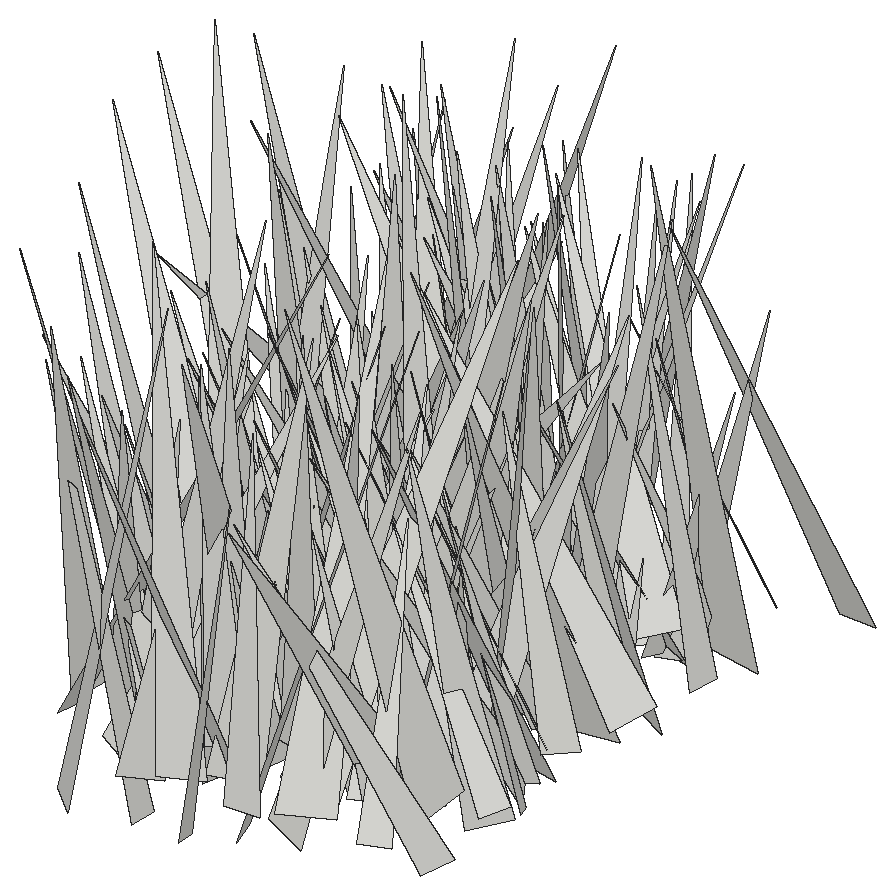
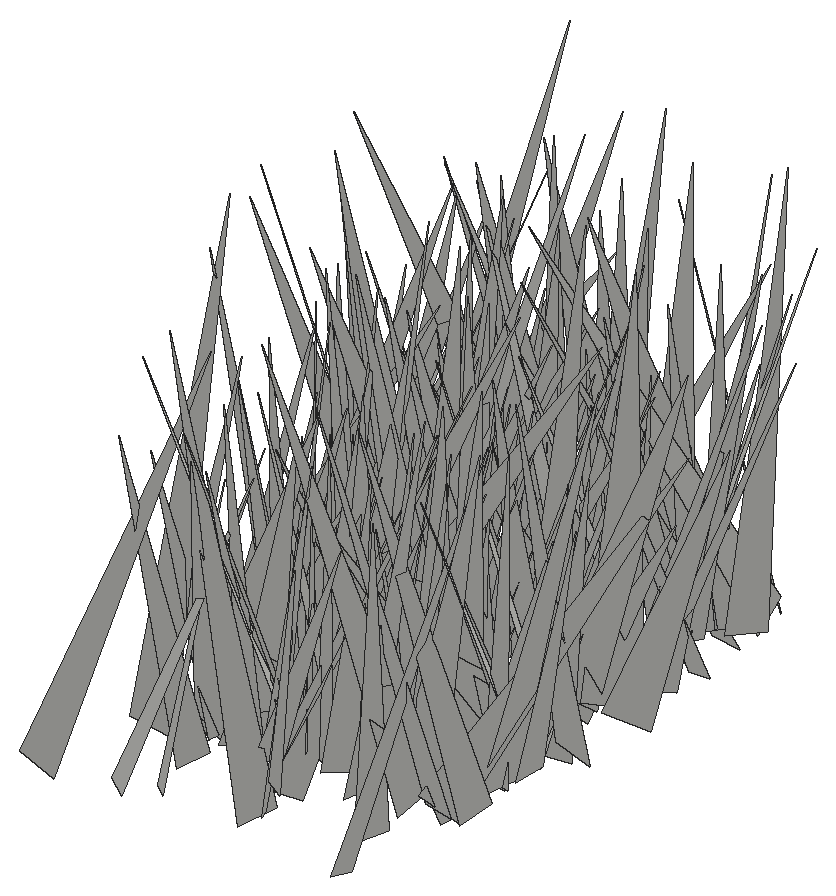
# SketchUp Ruby script. Lengths in inches.
U = 1.inch
M = Sketchup.active_model
def pt(a) = Geom::Point3d.new(a.map { |v| v * U })
def face(e, loops, mat)
  f = e.add_face(loops[0].map { |a| pt(a) })
  loops[1..].each { |l| e.add_face(l.map { |a| pt(a) }).erase! }
  f.material = f.back_material = mat if mat
  f
end
# faces: each face lists its corners as indices into pts; further lists are holes
def faces(e, pts, list, mat = nil) = list.each { |f| face(e, (f[0].is_a?(Array) ? f : [f]).map { |l| l.map { |i| pts[i] } }, mat) }
# xy, xz, yz: faces in a plane at the given z, y or x. An outline is a flat list of corners, or four numbers for a rectangle; further outlines are holes
def ring(l) = l.size == 4 ? [[l[0], l[1]], [l[2], l[1]], [l[2], l[3]], [l[0], l[3]]] : l.each_slice(2).to_a
def flat(e, list, mat, &to3) = list.each { |f| face(e, (f[0].is_a?(Array) ? f : [f]).map { |l| ring(l).map { |u, v| to3.(u, v) } }, mat) }
def xy(e, z, list, mat = nil) = flat(e, list, mat) { |x, y| [x, y, z] }
def xz(e, y, list, mat = nil) = flat(e, list, mat) { |x, z| [x, y, z] }
def yz(e, x, list, mat = nil) = flat(e, list, mat) { |y, z| [x, y, z] }
def lines(e, pts, list) = list.each { |a, b| e.add_line(pt(pts[a]), pt(pts[b])) }
# prism: a flat outline (further loops are holes) pulled along v
def prism(e, loops, v, mat = nil)
  f = face(e, loops, mat); d = Geom::Vector3d.new(v.map { |x| x * U })
  f.pushpull(f.normal.samedirection?(d) ? d.length : -d.length)
end
def box(e, o, s, mat = nil) = prism(e, [[o, [o[0] + s[0], o[1], o[2]], [o[0] + s[0], o[1] + s[1], o[2]], [o[0], o[1] + s[1], o[2]]]], [0, 0, s[2]], mat)
def at(x, y, z, deg = 0) = Geom::Transformation.translation(pt([x, y, z])) * Geom::Transformation.rotation(ORIGIN, Z_AXIS, deg.degrees)
def axes(o, x, y, z) = Geom::Transformation.new([*x, 0, *y, 0, *z, 0, *pt(o).to_a, 1])
def part(name) = M.definitions.add(name)
# library, detail: a bought-in or finely detailed component or shape, given as its bounding box
def library(name, o, s) = part(name).tap { |d| box(d.entities, o, s) }
def detail(e, o, s) = box(e.add_group.entities, o, s)
def put(e, d, t, mat = nil) = e.add_instance(d, t).tap { |i| i.material = mat if mat }
def group(e, t, mat = nil) = e.add_group.tap { |g| g.transformation = t; g.material = mat if mat }.entities
root = M.entities
c1 = part("fur_instance\#9")
p = [[0.8125,0,1.79],[0.67,-0.02,1.48],[0,-0.11,0],[0,0.11,0]]
faces(c1.entities,p,[[0,1,2,3]])
put(root,c1,axes([64.84,118.15,-27.1],[-3.24359,5.98487,0.42852],[5.75195,2.96279,2.1587],[-1.708,-1.38792,6.45597]))
put(root,c1,axes([65.26,123.43,-27.1],[-7.08698,0.49693,1.41438],[0.58095,7.2106,0.37757],[1.38199,-0.48283,7.09434]))
put(root,c1,axes([66.96,118.08,-27.1],[-3.17251,7.14398,0.8627],[6.87917,2.73438,2.65436],[-2.11131,-1.82544,7.35225]))
put(root,c1,axes([65.07,122.26,-27.1],[-4.79431,0.50788,0.77321],[0.45097,4.84644,-0.38709],[0.80772,0.30866,4.80557]))
put(root,c1,axes([65.85,125.42,-27.1],[3.04305,-5.48081,0.27728],[-4.42438,-2.6378,-3.58374],[-3.24669,-1.54241,5.14356]))
put(root,c1,axes([65.59,115.98,-27.1],[-5.22696,-1.19875,0.73288],[-0.94186,5.08442,1.59898],[1.04259,-1.41663,5.11873]))
put(root,c1,axes([65.69,117.69,-27.1],[-4.19179,6.94453,1.88873],[7.18228,4.17546,0.58769],[0.45687,-1.92457,8.09026]))
put(root,c1,axes([64.86,120.54,-27.1],[1.29784,6.7007,1.25957],[6.74597,-1.44798,0.75208],[-0.98888,-1.08363,6.78367]))
put(root,c1,axes([67.71,114.12,-28.22],[-7.51977,-1.08655,0.44758],[-1.14316,7.43533,-1.15625],[0.27218,1.20961,7.50937]))
put(root,c1,axes([67.67,117.16,-28.22],[-1.87407,5.07403,0.37598],[4.58214,1.50899,2.47512],[-2.21159,-1.17322,4.80954]))
put(root,c1,axes([65.07,116.1,-27.1],[-4.32761,-0.50237,2.11035],[0.41917,4.42689,1.9134],[2.12844,-1.89326,3.91401]))
put(root,c1,axes([66.42,113.57,-27.1],[-6.02827,1.48886,1.73676],[1.72693,6.17226,0.7029],[1.50026,-1.12234,6.1695]))
put(root,c1,axes([66.98,121.77,-28.22],[-1.60239,4.56784,1.22355],[4.62571,1.24567,1.40748],[-0.98238,-1.58525,4.63161]))
put(root,c1,axes([66.41,119.52,-28.22],[-2.06507,4.56305,1.47225],[4.79287,1.92061,0.77009],[-0.13147,-1.65628,4.94903]))
put(root,c1,axes([65.53,123.23,-27.1],[1.09401,4.63876,2.44173],[5.21296,-1.22556,-0.00737],[-0.55243,-2.37843,4.76601]))
put(root,c1,axes([67.625,111.83,-27.1],[-5.88104,-3.53705,0.94417],[-3.64814,5.81133,-0.9531],[0.30541,1.30636,6.79625]))
put(root,c1,axes([65.98,115.75,-27.1],[-3.08221,-2.2445,0.63722],[-2.14243,3.14072,0.69983],[0.92405,-0.20483,3.74807]))
put(root,c1,axes([66.2,121.26,-27.1],[3.80784,5.11048,0.67094],[4.57882,-3.73693,2.47721],[-2.36675,0.99257,5.87197]))
put(root,c1,axes([67.18,124.61,-27.1],[-2.59565,5.50063,1.7013],[5.74289,2.3395,1.19781],[-0.41302,-2.03926,5.96319]))
put(root,c1,axes([67.8,111.69,-27.1],[-4.98087,1.16288,0.32288],[1.15979,4.99131,-0.08543],[0.33384,0.00996,5.1141]))
put(root,c1,axes([65.36,112.02,-27.1],[6.33398,-2.31725,1.64534],[-1.9481,-6.46653,-1.60778],[-2.06922,-1.00519,6.55011]))
put(root,c1,axes([66.54,119.98,-28.22],[-3.71629,-3.62879,0.54604],[-3.4741,3.72939,1.13989],[1.18191,-0.44788,5.0675]))
put(root,c1,axes([64.92,114.73,-27.1],[1.35315,4.35582,0.79538],[4.34518,-1.14634,-1.11449],[0.85157,-1.07217,4.42291]))
put(root,c1,axes([66.9,128.53,-28.22],[-6.16239,-2.08969,1.53365],[-1.42213,6.03269,2.50561],[2.16712,-1.98337,6.00531]))
put(root,c1,axes([67.79,117.45,-27.1],[-4.13289,0.76106,0.51137],[0.79822,4.14817,0.27763],[0.45116,-0.36746,4.1932]))
put(root,c1,axes([64.83,125,-27.1],[6.22243,-0.20354,0.93497],[-0.30289,-6.25415,0.65425],[-0.90767,0.69164,6.19128]))
put(root,c1,axes([67.47,124.59,-27.1],[4.90342,0.51596,3.18153],[0.4361,-5.84514,0.27581],[-3.19346,-0.00597,4.92277]))
put(root,c1,axes([68.41,122.6875,-28.22],[-6.24341,4.5177,1.05822],[4.50521,6.32678,-0.4296],[1.11019,-0.26807,7.69449]))
put(root,c1,axes([66.2,112.4,-27.1],[5.00192,-1.81934,1.03799],[-1.65,-5.07776,-0.94895],[-1.29032,-0.55947,5.23724]))
put(root,c1,axes([67.18,119.29,-28.22],[-0.06707,-7.91469,2.47451],[-8.29222,0.04381,-0.08466],[-0.06773,2.47503,7.91452]))
put(root,c1,axes([68.17,126.02,-27.1],[-6.22894,0.57755,1.75246],[0.68588,6.45268,0.31131],[1.71297,-0.48351,6.24791]))
put(root,c1,axes([66.53,112.71,-27.1],[6.05103,1.03829,2.78411],[2.19851,-5.8136,-2.61017],[-1.99898,-3.2509,5.55698]))
put(root,c1,axes([69.5,108.86,-28.22],[-6.22819,-1.34042,0.61243],[-1.44458,6.07908,-1.38568],[0.29149,1.48668,6.21828]))
put(root,c1,axes([68.08,118.91,-28.22],[-5.34659,-1.99732,0.9572],[-1.60106,5.21354,1.93576],[1.5304,-1.52357,5.36919]))
put(root,c1,axes([65.77,125.51,-27.1],[2.77668,6.00015,1.42785],[6.14966,-2.57364,-1.14395],[0.47149,-1.76779,6.51177]))
put(root,c1,axes([67.5625,126.33,-28.22],[-4.75498,1.70819,1.94206],[1.76287,5.11453,-0.18234],[1.89256,-0.47231,5.04921]))
put(root,c1,axes([68.23,116.49,-27.1],[-3.61922,1.27993,0.57976],[1.16278,3.62754,-0.74965],[0.78884,0.52519,3.76496]))
put(root,c1,axes([66.6,112.66,-27.1],[2.66304,-4.00114,1.09323],[-4.14622,-2.60379,0.57024],[-0.11461,1.22768,4.77239]))
put(root,c1,axes([67.33,124.14,-27.1],[-1.25475,3.57203,1.31412],[3.70812,1.4592,-0.42579],[0.858,-1.08261,3.76198]))
put(root,c1,axes([70.04,118.73,-28.22],[-4.54723,-4.75664,0.92618],[-4.80738,4.26788,-1.68375],[-0.61038,1.82216,6.36144]))
put(root,c1,axes([67.2,119.92,-28.22],[3.79033,1.52401,0.8214],[1.29616,-3.80865,1.0854],[-1.14773,0.73179,3.93842]))
put(root,c1,axes([68.78,120.83,-27.1],[3.00603,-4.02582,3.59921],[-4.80148,-3.87769,-0.32715],[-2.47129,2.63706,5.01362]))
put(root,c1,axes([67.25,108.29,-28.22],[4.64173,5.41011,1.53464],[5.42173,-4.8336,0.64123],[-1.49305,-0.73288,7.09956]))
put(root,c1,axes([67.07,113.09,-28.22],[2.82826,-4.43632,2.67471],[-5.15951,-2.68482,1.00262],[-0.46309,2.81866,5.16476]))
put(root,c1,axes([65.51,110.8,-27.1],[7.33228,1.89466,0.16833],[1.78282,-7.07911,2.02191],[-0.66303,1.91751,7.29821]))
put(root,c1,axes([67.9375,118.45,-27.1],[-1.16882,5.10436,1.64073],[5.31118,1.33199,-0.3603],[0.7334,-1.51127,5.22406]))
put(root,c1,axes([68.32,125.61,-28.22],[-5.67591,-0.59927,2.29984],[-0.30227,6.08824,0.84044],[2.35734,-0.66225,5.64524]))
put(root,c1,axes([69.52,119.3125,-27.1],[-0.27528,4.26527,0.41219],[4.05575,0.12601,1.40472],[-1.38323,-0.47937,4.03672]))
put(root,c1,axes([67.23,124.49,-27.1],[1.7878,3.1828,1.34143],[3.44443,-1.53093,-0.95817],[0.2561,-1.62848,3.52255]))
put(root,c1,axes([67.1875,114.24,-28.22],[5.06961,3.19969,0.78256],[3.08145,-5.11429,0.94868],[-1.16407,0.39664,5.91937]))
put(root,c1,axes([72.34,121.27,-27.1],[-3.051,-7.21191,1.32168],[-6.61753,2.09219,-3.8598],[-3.15701,2.58422,6.81338]))
put(root,c1,axes([69.63,111.6,-28.22],[-5.24858,-0.93793,1.2858],[-1.33069,5.01688,-1.77222],[0.87308,2.00792,5.02857]))
put(root,c1,axes([69.12,120.68,-28.22],[-5.6995,-3.45113,0.56108],[-3.05969,5.44221,2.39374],[1.69215,-1.78365,6.21808]))
put(root,c1,axes([67.03,121.89,-27.1],[-1.28039,5.01222,0.36244],[4.5705,1.31696,-2.06622],[2.08908,0.19072,4.74262]))
put(root,c1,axes([68.97,123.79,-27.1],[3.31439,2.62679,2.62231],[3.03004,-3.94532,0.12232],[-2.14367,-1.5153,4.22732]))
put(root,c1,axes([66.57,119.5625,-27.1],[4.70564,3.18962,0.73071],[3.27223,-4.59158,-1.02983],[-0.01227,-1.26267,5.59072]))
put(root,c1,axes([70.63,117.9375,-28.22],[-2.19806,-5.17129,0.07017],[-4.98418,2.09779,-1.52836],[-1.38027,0.66005,5.4072]))
put(root,c1,axes([68.04,121.0625,-28.22],[-4.86484,4.13925,3.64162],[4.78109,5.5858,0.03796],[2.74517,-2.39309,6.38738]))
put(root,c1,axes([66.61,125.52,-27.1],[7.58645,0.4489,1.20084],[0.2907,-7.62155,1.01257],[-1.24861,0.95304,7.53196]))
put(root,c1,axes([69.76,115.34,-28.22],[-6.59248,-1.12335,1.64682],[-1.04061,6.79216,0.46743],[1.70031,-0.1986,6.67115]))
put(root,c1,axes([68.28,120.45,-27.1],[4.10212,-1.60455,0.85508],[-1.23063,-4.00368,-1.60913],[-1.3384,-1.23658,4.10033]))
put(root,c1,axes([66.73,111.22,-28.22],[2.4491,6.4359,0.09226],[6.32974,-2.3903,-1.28384],[1.16776,-0.54137,6.7654]))
put(root,c1,axes([71.85,125.07,-28.22],[-7.66892,-1.90839,0.15613],[-1.91216,7.66661,-0.21311],[0.09999,0.24454,7.89993]))
put(root,c1,axes([70.18,109.5625,-27.1],[-1.69454,7.12423,1.83382],[7.32335,1.45532,1.11334],[-0.69716,-2.02889,7.23786]))
put(root,c1,axes([70.8,117.98,-27.1],[-4.9286,0.63717,0.02707],[0.62924,4.89286,-0.60144],[0.10377,0.59304,4.93308]))
put(root,c1,axes([69.33,108.95,-27.1],[-6.96616,2.88196,1.8212],[2.05018,6.85162,-3.00033],[2.72382,2.21349,6.91601]))
put(root,c1,axes([71.57,110.26,-27.1],[-3.32714,-4.87132,0.7615],[-4.7527,2.92423,-2.05917],[-1.31203,1.7603,5.52806]))
put(root,c1,axes([70.46,123.27,-28.22],[0.69444,-4.60057,1.02449],[-4.36557,-1.0182,-1.61314],[-1.77671,0.70364,4.36409]))
put(root,c1,axes([69.4,125.52,-27.1],[-3.39336,2.50243,2.08506],[2.97495,3.60715,0.51243],[1.32637,-1.68843,4.18502]))
put(root,c1,axes([66.8125,120.625,-28.22],[5.86888,-2.59714,0.14419],[-2.59865,-5.83866,0.60558],[0.11385,0.61201,6.38922]))
put(root,c1,axes([69.11,116.08,-28.22],[3.19373,2.97376,0.94617],[2.91746,-3.32577,0.60507],[-1.10768,-0.18543,4.3217]))
put(root,c1,axes([67.9,114.83,-28.22],[-0.42992,-4.68733,0.89248],[-4.33891,0.75688,1.88505],[1.98531,0.63912,4.31306]))
put(root,c1,axes([72.78,121.91,-27.1],[-6.95314,3.37085,0.59923],[3.40426,6.66259,2.02209],[-0.36434,-2.07731,7.45788]))
put(root,c1,axes([71.16,125.97,-28.22],[3.15853,-4.87453,2.05329],[-4.28659,-3.76007,-2.33247],[-3.09874,0.23284,5.31949]))
put(root,c1,axes([71.38,126.27,-27.1],[-4.19942,1.95994,0.17006],[1.96728,4.18576,0.33862],[0.01038,-0.37878,4.62189]))
put(root,c1,axes([71.82,123.75,-28.22],[-5.34119,3.3335,0.99515],[3.47843,5.14626,1.43085],[0.05516,-1.74201,6.13133]))
put(root,c1,axes([70.14,111.66,-27.1],[1.65081,-5.08845,2.41171],[-5.51574,-1.96719,-0.37505],[-1.13372,2.16141,5.33637]))
put(root,c1,axes([68.52,115.18,-28.22],[7.11754,-4.23376,0.53848],[-3.90576,-6.88369,-2.49681],[-1.7204,-1.88792,7.89621]))
put(root,c1,axes([71.87,122.33,-28.22],[-2.19401,4.08598,0.64459],[3.98986,1.89782,1.55038],[-1.09165,-1.27572,4.37096]))
put(root,c1,axes([70.47,119.62,-27.1],[0.64716,8.27924,1.09317],[8.31403,-0.74193,0.69715],[-0.78591,-1.0312,8.27518]))
put(root,c1,axes([66.4,123.8,-28.22],[2.58062,-5.27777,0.62862],[-4.46822,-1.77579,3.43383],[2.87837,1.97518,4.76689]))
put(root,c1,axes([70.23,127.41,-27.1],[-1.89592,-3.45095,1.30694],[-3.60556,2.04518,0.16982],[0.78554,1.05823,3.9338]))
put(root,c1,axes([69.74,112.5,-27.1],[2.04038,-5.82637,1.87095],[-6.1057,-2.07021,0.21174],[-0.4092,1.83789,6.16967]))
put(root,c1,axes([70.04,125.37,-27.1],[-2.18081,-4.36379,1.96245],[-4.63729,2.45895,0.31456],[1.17875,1.60022,4.86823]))
put(root,c1,axes([71.23,125.05,-28.22],[-3.89073,-3.2521,0.98713],[-3.3181,3.95947,-0.03367],[0.73538,0.65937,5.07078]))
put(root,c1,axes([70.78,119.67,-27.1],[-3.9819,-2.09854,0.99873],[-1.89028,4.07705,1.03024],[1.35209,-0.4803,4.38155]))
put(root,c1,axes([68.3,120.58,-27.1],[3.9818,-4.86666,0.84742],[-4.90357,-3.76221,1.43455],[0.59785,1.55519,6.12218]))
put(root,c1,axes([71.84,122.3,-28.22],[-6.35948,3.06032,1.72749],[3.24757,6.48259,0.47123],[1.34279,-1.18457,7.04176]))
put(root,c1,axes([71.05,124.27,-27.1],[1.22573,-5.85041,2.29876],[-6.17569,-1.55733,-0.67049],[-1.1715,2.08841,5.93971]))
put(root,c1,axes([68.97,114.5,-28.22],[0.04423,5.29855,0.55334],[5.02486,0.14232,-1.76445],[1.76963,-0.53655,4.99632]))
put(root,c1,axes([72.18,121.26,-28.22],[-6.55915,2.85076,0.80174],[2.70921,6.56329,-1.17278],[1.19574,0.76707,7.05506]))
put(root,c1,axes([72.45,117.34,-27.1],[0.0482,8.00911,1.76337],[7.92916,-0.49572,2.03478],[-2.09374,-1.69294,7.74648]))
put(root,c1,axes([72.39,124.66,-27.1],[-5.98582,-0.44068,0.88109],[-0.67667,5.78235,-1.70504],[0.71598,1.78068,5.75475]))
put(root,c1,axes([70.42,113.36,-28.22],[3.22144,-2.0672,0.86258],[-1.86043,-3.31076,-0.98626],[-1.24746,-0.40075,3.69841]))
put(root,c1,axes([72.33,113.7,-27.1],[-3.83694,1.86592,0.39498],[1.90547,3.78872,0.61201],[0.08273,-0.72368,4.22246]))
put(root,c1,axes([71.05,108.71,-28.22],[-4.14484,-0.82966,2.07391],[-1.4546,4.32013,-1.17886],[1.69516,1.67847,4.05935]))
put(root,c1,axes([68.45,115.64,-27.1],[6.75177,1.95337,0.7466],[2.07523,-6.56983,-1.57805],[-0.25785,-1.72661,6.84922]))
put(root,c1,axes([70.91,126.88,-28.22],[6.14406,2.36607,3.59044],[3.36505,-6.54408,-1.44586],[-2.67694,-2.79567,6.42319]))
put(root,c1,axes([70.68,124.26,-27.1],[-2.8459,-6.01928,1.64103],[-5.98512,3.14324,1.14988],[1.76154,0.95508,6.5581]))
put(root,c1,axes([70.82,123.12,-28.22],[3.4639,-0.21189,1.20284],[0.06017,-3.58323,-0.80448],[-1.21988,-0.7784,3.37584]))
put(root,c1,axes([72.65,115.47,-28.22],[2.36274,4.29484,1.97791],[3.91667,-3.01643,1.87116],[-2.64906,-0.62918,4.53067]))
put(root,c1,axes([72.46,120.21,-27.1],[-0.70477,-3.63934,0.22038],[-3.52996,0.62491,-0.96896],[-0.91253,0.39339,3.57807]))
put(root,c1,axes([71.25,113.46,-28.22],[3.09242,2.58599,1.68004],[2.84079,-3.31463,-0.12697],[-1.19992,-1.18273,4.02918]))
put(root,c1,axes([70.28,124.28,-27.1],[5.04239,2.3615,1.06864],[2.46365,-5.09289,-0.37039],[-0.80566,-0.79378,5.55564]))
put(root,c1,axes([73.37,119,-27.1],[-7.60319,-2.30719,2.08818],[-2.71089,7.61771,-1.45385],[1.52798,2.03457,7.8114]))
put(root,c1,axes([70.53,116.51,-27.1],[3.48298,2.03603,0.22687],[2.02285,-3.48877,0.25421],[-0.32396,0.10555,4.02641]))
put(root,c1,axes([72.23,113.2,-27.1],[-4.31803,3.62073,2.04082],[3.93255,4.51165,0.31626],[1.34522,-1.56695,5.62628]))
put(root,c1,axes([73.69,124.02,-28.22],[-5.31881,4.24046,0.31909],[4.24772,5.322,0.07866],[0.20039,-0.26047,6.80184]))
put(root,c1,axes([70.6875,115.49,-28.22],[3.85375,-0.57416,0.66525],[-0.65849,-3.86826,0.47595],[-0.58191,0.57487,3.8671]))
put(root,c1,axes([71,124.84,-27.1],[5.57047,2.74276,2.66238],[3.42235,-5.67452,-1.31471],[-1.7025,-2.43273,6.06831]))
put(root,c1,axes([71.38,122.86,-27.1],[2.3019,2.88607,2.09295],[3.52279,-2.224,-0.8077],[-0.54756,-2.17555,3.60219]))
put(root,c1,axes([73.53,119.46,-27.1],[-3.08913,-1.9262,0.20442],[-1.91689,2.98464,-0.84391],[-0.27849,0.82245,3.5413]))
put(root,c1,axes([71.76,116.8,-28.22],[-2.01295,-3.23513,0.63988],[-3.06607,2.112,1.03257],[1.21439,-0.03018,3.66768]))
put(root,c1,axes([73.74,124.52,-28.22],[-5.02266,3.34128,1.54054],[3.64584,4.87057,1.32283],[0.49523,-1.96924,5.88569]))
put(root,c1,axes([71.34,110.43,-27.1],[-3.27295,5.40819,2.7555],[5.57889,3.91368,-1.05481],[2.39109,-1.7286,6.23283]))
put(root,c1,axes([74.11,115,-27.1],[-4.51711,1.79985,0.33219],[1.82954,4.41557,0.95372],[-0.05124,-1.00862,4.76803]))
put(root,c1,axes([71.75,112.7,-27.1],[-0.58668,-6.43534,2.37936],[-6.81319,0.82822,0.56013],[0.80964,2.30643,6.43771]))
put(root,c1,axes([73.1875,116.55,-28.22],[-3.55756,1.9012,0.49829],[1.88183,3.59228,-0.2708],[0.56709,0.00632,4.02461]))
put(root,c1,axes([72.57,109.22,-27.1],[-0.09344,5.23116,1.72248],[5.50098,0.0052,0.28262],[-0.26677,-1.725,5.22436]))
put(root,c1,axes([71.47,124.76,-27.1],[3.13584,4.70476,0.63652],[4.72939,-3.16238,0.0748],[-0.41563,-0.48786,5.65355]))
put(root,c1,axes([69.64,120.56,-27.1],[3.88235,-7.18309,1.19208],[-7.15051,-3.50623,2.16032],[1.37403,2.04942,7.87416]))
put(root,c1,axes([72.84,113.82,-28.22],[-3.68775,-0.43694,1.2324],[0.03671,3.65173,1.40455],[1.30705,-1.33536,3.43768]))
put(root,c1,axes([75.02,114.47,-28.22],[-3.41079,-4.86692,0.40111],[-4.72199,3.16213,-1.78467],[-1.24525,1.33989,5.66881]))
put(root,c1,axes([72.66,115.1875,-27.1],[4.91626,-1.03874,2.91243],[-2.03601,-5.20453,1.58061],[-2.3272,2.35896,4.76972]))
put(root,c1,axes([73.25,117.44,-28.22],[-3.81436,-7.20009,0.2192],[-7.12697,3.80817,1.069],[1.0467,-0.30859,8.07762]))
put(root,c1,axes([71.92,121.53,-27.1],[2.13967,5.72529,2.72362],[6.33838,-1.99885,-0.77766],[-0.14822,-2.82858,6.06237]))
put(root,c1,axes([75.21,123.56,-27.1],[-4.13597,4.87198,0.25098],[4.78591,3.98836,1.44689],[-0.94567,-1.12348,6.22487]))
put(root,c1,axes([70.82,127.45,-28.22],[7.358,-0.55238,1.16955],[-0.51092,-7.44716,-0.30295],[-1.18825,-0.21839,7.37248]))
put(root,c1,axes([71.35,116.09,-28.22],[4.05743,2.55482,1.17911],[2.80714,-3.81746,-1.3882],[-0.19333,-1.81108,4.58942]))
put(root,c1,axes([71.5,114.37,-27.1],[5.97247,-1.71505,1.0533],[-1.60325,-6.04797,-0.7569],[-1.21673,-0.44932,6.16757]))
put(root,c1,axes([72.42,116.28,-27.1],[5.48977,-0.87036,1.92832],[-0.64898,-5.79667,-0.76876],[-2.01365,-0.50463,5.50492]))
put(root,c1,axes([73.16,114.94,-28.22],[2.88206,-3.90926,2.29022],[-4.22914,-3.29495,-0.30223],[-1.62535,1.64154,4.8474]))
put(root,c1,axes([72.87,125.08,-28.22],[1.59622,5.71911,2.00108],[6.0184,-1.73595,0.16062],[-0.70101,-1.88115,5.93551]))
put(root,c1,axes([73.65,113.32,-28.22],[-3.2921,4.67046,0.35788],[4.62081,3.30978,-0.68745],[0.76768,0.10645,5.67261]))
put(root,c1,axes([71.93,117.0625,-27.1],[6.32729,-2.1008,2.73388],[-3.01636,-6.1404,2.26257],[-1.67006,3.13117,6.27127]))
put(root,c1,axes([73.9,122.35,-27.1],[1.51119,6.34193,0.92742],[6.21067,-1.68435,1.39797],[-1.58356,-0.55387,6.36784]))
put(root,c1,axes([75.16,114.9,-28.22],[-4.72001,4.32069,1.36462],[4.52973,4.45158,1.57294],[-0.11027,-2.07946,6.20264]))
put(root,c1,axes([75.23,116.87,-27.1],[-1.27036,4.00789,0.19304],[3.62684,1.0603,1.85365],[-1.71652,-0.72583,3.77372]))
put(root,c1,axes([72.76,118.65,-27.1],[-3.43989,-5.36661,0.1848],[-4.97328,3.26677,2.29397],[2.02515,-1.09328,5.94736]))
put(root,c1,axes([71.37,125.22,-28.22],[6.23542,-1.61716,0.46655],[-1.48447,-6.12774,-1.40019],[-0.79324,-1.24458,6.2877]))
put(root,c1,axes([74.64,122.53,-28.22],[1.87355,6.48838,0.26131],[6.01197,-1.83596,2.48253],[-2.45429,0.45575,6.28063]))
put(root,c1,axes([74.16,114.33,-28.22],[-6.37075,2.32719,2.17346],[2.54476,6.64308,0.34616],[1.91413,-1.08621,6.77365]))
put(root,c1,axes([72.08,109.89,-28.22],[6.70956,3.50603,1.11128],[3.28027,-6.75003,1.49074],[-1.66343,0.8308,7.42214]))
put(root,c1,axes([75.27,124.36,-28.22],[-2.21504,-4.22644,0.02495],[-4.06696,2.12371,-1.31133],[-1.15036,0.62998,4.58799]))
put(root,c1,axes([74.07,110.06,-27.1],[-5.45003,5.37343,0.92209],[5.18096,5.51046,-1.48977],[1.69756,0.43353,7.50714]))
put(root,c1,axes([74.02,121.42,-28.22],[-4.28655,1.17606,1.86698],[1.8295,4.17484,1.57066],[1.23356,-2.10497,4.15821]))
put(root,c1,axes([71.85,124.61,-27.1],[4.96936,4.425,0.65774],[4.44372,-4.99597,0.03757],[-0.51632,-0.4092,6.65385]))
put(root,c1,axes([72.27,121.6,-27.1],[1.6892,-5.96403,1.00433],[-6.01842,-1.55459,0.89085],[0.59746,1.20222,6.13428]))
put(root,c1,axes([75.07,124.27,-28.22],[1.09357,6.43106,0.77169],[6.11568,-1.28298,2.02542],[-2.13365,-0.38127,6.20097]))
put(root,c1,axes([72.22,123.04,-27.1],[-0.71595,-3.844,0.50308],[-3.36107,0.87042,1.86752],[1.93201,0.08975,3.4353]))
put(root,c1,axes([72.93,115.3,-27.1],[2.99625,3.60782,0.19235],[3.59342,-3.00177,0.328],[-0.37513,0.06212,4.67828]))
put(root,c1,axes([75.04,128.55,-28.22],[-3.18461,-4.17271,0.10236],[-4.17132,3.18622,0.10881],[0.1486,0.01532,5.24799]))
put(root,c1,axes([73.94,127.96,-28.22],[-3.11173,-3.4795,0.92655],[-3.33661,3.24675,0.98692],[1.3537,0.0043,4.56244]))
put(root,c1,axes([72.06,118.92,-27.1],[4.17452,-5.37379,1.20818],[-5.50555,-4.02647,1.11376],[0.16212,1.6352,6.71296]))
put(root,c1,axes([74.75,112.51,-28.22],[-4.43499,0.78648,1.49873],[1.10021,4.53377,0.87655],[1.28619,-1.16631,4.41807]))
put(root,c1,axes([74.12,119.49,-28.22],[-0.34138,-6.1128,0.75859],[-6.1403,0.39794,0.44341],[0.48829,0.7305,6.10625]))
put(root,c1,axes([76.03,117.8,-27.1],[0.12283,-4.44104,1.09952],[-4.1986,-0.54638,-1.73783],[-1.81756,0.96203,4.08875]))
put(root,c1,axes([77.55,119.5625,-27.1],[-6.03456,2.61232,0.13904],[2.52964,5.73798,1.98392],[-0.66667,-1.87372,6.2693]))
put(root,c1,axes([73.01,110.5,-28.22],[2.20928,6.37096,1.50715],[6.50914,-1.9672,-1.22586],[0.70121,-1.81177,6.63078]))
put(root,c1,axes([76.12,119.8,-28.22],[-0.98604,-7.77609,1.14314],[-7.75331,0.77346,-1.42635],[-1.28859,1.29646,7.70749]))
put(root,c1,axes([77.14,115.42,-28.22],[-5.24793,-3.08562,0.82091],[-3.15493,4.76816,-2.24651],[-0.49124,2.34081,5.65818]))
put(root,c1,axes([74.94,122.1,-27.1],[3.15907,-2.58161,1.45094],[-2.40771,-3.47422,-0.93937],[-1.72421,0.12146,3.97014]))
put(root,c1,axes([74.52,113.89,-28.22],[6.08431,-4.17162,0.61258],[-3.3903,-5.47976,-3.64343],[-2.50671,-2.71408,6.41457]))
put(root,c1,axes([73.3,111.16,-27.1],[-0.97355,8.05143,1.14446],[7.84551,1.23329,-2.00251],[2.14086,-0.85824,7.85896]))
put(root,c1,axes([73.89,116.83,-28.22],[1.68223,-3.64936,0.16027],[-3.63941,-1.65928,0.41825],[0.31341,0.31999,3.9966]))
put(root,c1,axes([73.4,122.7,-27.1],[2.35807,6.09522,2.44102],[6.53945,-1.94795,-1.45322],[0.58808,-2.77931,6.37184]))
put(root,c1,axes([76.66,116.97,-27.1],[-2.71564,-2.49022,0.0198],[-2.39499,2.6036,-1.03032],[-0.68234,0.77224,3.53756]))
put(root,c1,axes([74.78,113.17,-27.1],[4.77639,3.07128,1.21309],[2.81816,-4.90311,1.31748],[-1.72115,0.49496,5.52367]))
put(root,c1,axes([75.84,124.91,-27.1],[-3.61169,-1.5954,0.61372],[-1.41522,3.59542,1.01805],[0.9587,-0.70282,3.81487]))
put(root,c1,axes([76.1,117.36,-28.22],[-1.51656,-6.50321,0.08888],[-6.50028,1.51258,-0.24097],[-0.21452,0.14123,6.67335]))
put(root,c1,axes([76.29,116.51,-28.22],[-5.86145,-3.99032,0.23805],[-3.68658,5.55942,2.41617],[1.54546,-1.87245,6.66644]))
put(root,c1,axes([76.58,112.59,-27.1],[-7.9399,0.37328,2.34081],[0.92834,8.01881,1.87016],[2.18103,-2.05426,7.72553]))
put(root,c1,axes([74.29,126.01,-28.22],[4.97792,-1.2009,1.19397],[-1.36113,-5.04298,0.6026],[-1.0075,0.87956,5.08515]))
put(root,c1,axes([78.51,110.09,-27.1],[-2.5232,4.5633,1.53247],[4.25008,1.29942,3.12842],[-2.26029,-2.65076,4.17172]))
put(root,c1,axes([72.17,118.02,-28.22],[6.41393,4.45568,0.74677],[4.39818,-5.86174,-2.80093],[1.0328,-2.70854,7.29015]))
put(root,c1,axes([75,116.86,-28.22],[6.28919,2.00514,2.27548],[2.25266,-6.59596,-0.4138],[-2.03074,-1.10685,6.58812]))
put(root,c1,axes([76.23,116.63,-28.22],[0.87067,-3.63818,0.96208],[-3.64876,-1.05785,-0.69825],[-0.92116,0.75142,3.67517]))
put(root,c1,axes([74.61,124.25,-28.22],[4.30722,-1.10997,0.82887],[-1.21703,-4.32511,0.53238],[-0.66174,0.72977,4.41597]))
put(root,c1,axes([76.47,109.96,-27.1],[-1.50833,4.20798,0.27956],[4.21722,1.50618,0.08227],[0.01672,-0.29093,4.46939]))
put(root,c1,axes([77.83,113.35,-27.1],[-3.1989,2.68909,0.37978],[2.66785,3.00183,1.21655],[-0.50792,-1.16886,3.99802]))
put(root,c1,axes([77.61,128.98,-28.22],[-1.54524,-6.7658,0.51217],[-6.71547,1.44992,-1.10738],[-0.96994,0.74015,6.85109]))
put(root,c1,axes([77.2,116.9375,-27.1],[1.69917,-3.99461,2.49122],[-4.30676,-2.38859,-0.89256],[-1.90128,1.84064,4.24822]))
put(root,c1,axes([76.43,125.23,-28.22],[-1.19832,-8.06423,2.00487],[-8.30399,1.23724,0.01324],[0.30817,1.98109,8.15276]))
put(root,c1,axes([74.62,115.9,-28.22],[-0.40245,7.17423,1.83924],[7.10701,0.89237,-1.92572],[2.08393,-1.65784,6.92265]))
put(root,c1,axes([76.91,114.3,-28.22],[3.86572,-4.28586,2.24353],[-4.19582,-4.39988,-1.17556],[-2.40771,0.7863,5.6507]))
put(root,c1,axes([77.86,122.14,-27.1],[-5.58164,-0.15602,0.84627],[-0.25003,5.60842,-0.61509],[0.82341,0.64537,5.54984]))
put(root,c1,axes([76.86,121.22,-28.22],[-2.33347,-4.94017,0.88075],[-4.99474,2.38012,0.11709],[0.48332,0.74554,5.4623]))
